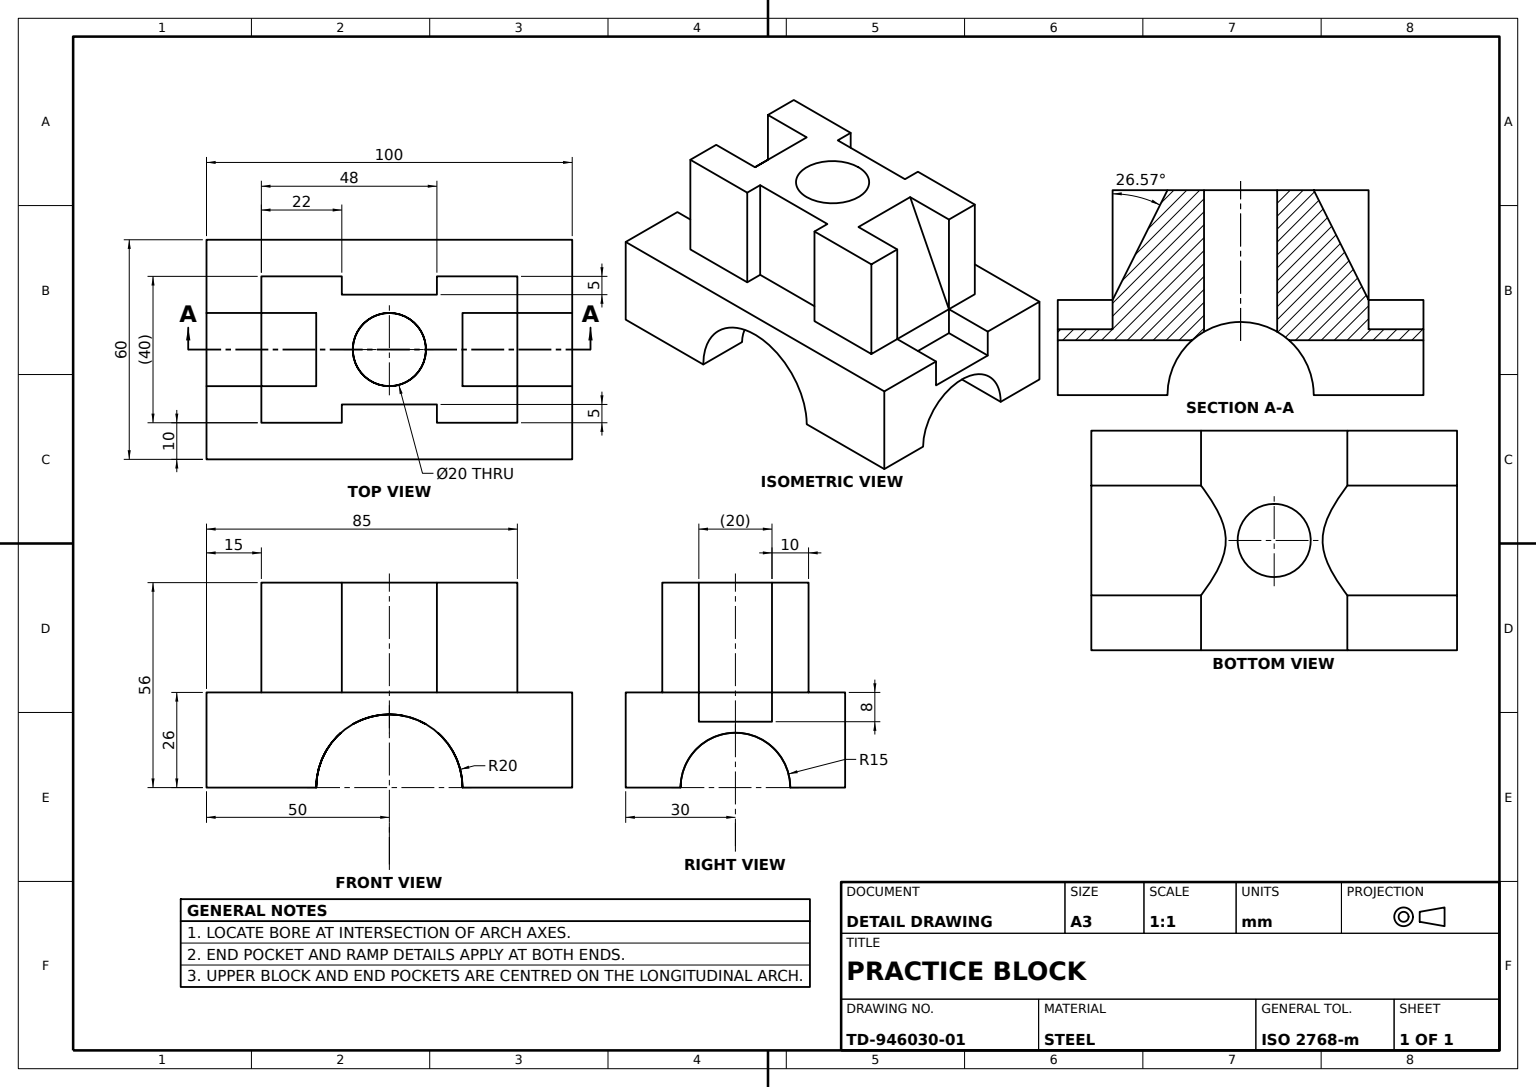
ISO-10303-21;
HEADER;
FILE_DESCRIPTION((''),'2;1');
FILE_NAME('','',(''),(''),'','','');
FILE_SCHEMA(('AUTOMOTIVE_DESIGN'));
ENDSEC;
DATA;
#1=APPLICATION_CONTEXT('');
#2=PRODUCT_CONTEXT('',#1,'mechanical');
#3=PRODUCT('','','',(#2));
#4=PRODUCT_DEFINITION_FORMATION('','',#3);
#5=PRODUCT_DEFINITION_CONTEXT('',#1,'design');
#6=PRODUCT_DEFINITION('','',#4,#5);
#7=PRODUCT_DEFINITION_SHAPE('','',#6);
#8=(LENGTH_UNIT()NAMED_UNIT(*)SI_UNIT(.MILLI.,.METRE.));
#9=(NAMED_UNIT(*)PLANE_ANGLE_UNIT()SI_UNIT($,.RADIAN.));
#10=(NAMED_UNIT(*)SI_UNIT($,.STERADIAN.)SOLID_ANGLE_UNIT());
#11=UNCERTAINTY_MEASURE_WITH_UNIT(LENGTH_MEASURE(1.E-05),#8,'distance_accuracy_value','');
#12=(GEOMETRIC_REPRESENTATION_CONTEXT(3)GLOBAL_UNCERTAINTY_ASSIGNED_CONTEXT((#11))GLOBAL_UNIT_ASSIGNED_CONTEXT((#8,#9,#10))REPRESENTATION_CONTEXT('',''));
#13=CARTESIAN_POINT('',(-20.,0.,15.));
#14=VERTEX_POINT('',#13);
#15=CARTESIAN_POINT('',(-20.,0.,30.));
#16=VERTEX_POINT('',#15);
#17=CARTESIAN_POINT('',(-20.,0.,91.));
#18=DIRECTION('',(0.,0.,1.));
#19=VECTOR('',#18,1000.);
#20=LINE('',#17,#19);
#21=EDGE_CURVE('',#14,#16,#20,.T.);
#22=ORIENTED_EDGE('',*,*,#21,.F.);
#23=CARTESIAN_POINT('',(-20.,0.,-15.));
#24=VERTEX_POINT('',#23);
#25=CARTESIAN_POINT('',(-20.,1.039988,-15.));
#26=CARTESIAN_POINT('',(-19.91945,2.055511,-14.89307));
#27=CARTESIAN_POINT('',(-19.68971,3.545099,-14.583876));
#28=CARTESIAN_POINT('',(-19.594347,4.038167,-14.455074));
#29=CARTESIAN_POINT('',(-19.370481,5.00297,-14.150132));
#30=CARTESIAN_POINT('',(-19.243229,5.47024,-13.975697));
#31=CARTESIAN_POINT('',(-18.961995,6.377158,-13.585856));
#32=CARTESIAN_POINT('',(-18.807998,6.816797,-13.37044));
#33=CARTESIAN_POINT('',(-18.476456,7.670078,-12.899895));
#34=CARTESIAN_POINT('',(-18.297983,8.085575,-12.64341));
#35=CARTESIAN_POINT('',(-17.739419,9.278133,-11.825632));
#36=CARTESIAN_POINT('',(-17.337061,10.001911,-11.218166));
#37=CARTESIAN_POINT('',(-16.711435,10.994586,-10.214717));
#38=CARTESIAN_POINT('',(-16.498395,11.31093,-9.863302));
#39=CARTESIAN_POINT('',(-16.073156,11.907469,-9.134223));
#40=CARTESIAN_POINT('',(-15.861739,12.18674,-8.758001));
#41=CARTESIAN_POINT('',(-15.238528,12.970461,-7.592364));
#42=CARTESIAN_POINT('',(-14.836864,13.421647,-6.766908));
#43=CARTESIAN_POINT('',(-14.29593,13.989091,-5.434909));
#44=CARTESIAN_POINT('',(-14.125386,14.160451,-4.972426));
#45=CARTESIAN_POINT('',(-13.822168,14.456576,-4.031229));
#46=CARTESIAN_POINT('',(-13.688686,14.582271,-3.550951));
#47=CARTESIAN_POINT('',(-13.467259,14.78701,-2.568307));
#48=CARTESIAN_POINT('',(-13.379218,14.866168,-2.065023));
#49=CARTESIAN_POINT('',(-13.259474,14.973069,-1.036579));
#50=CARTESIAN_POINT('',(-13.22921,14.9996,-0.523513));
#51=CARTESIAN_POINT('',(-13.228313,15.000391,0.500332));
#52=CARTESIAN_POINT('',(-13.257676,14.974649,1.011111));
#53=CARTESIAN_POINT('',(-13.374088,14.870772,2.030418));
#54=CARTESIAN_POINT('',(-13.461925,14.791862,2.540716));
#55=CARTESIAN_POINT('',(-13.682828,14.587763,3.528684));
#56=CARTESIAN_POINT('',(-13.816081,14.462383,4.010379));
#57=CARTESIAN_POINT('',(-14.118367,14.167438,4.952509));
#58=CARTESIAN_POINT('',(-14.288407,13.996778,5.415214));
#59=CARTESIAN_POINT('',(-14.829898,13.429354,6.752021));
#60=CARTESIAN_POINT('',(-15.232138,12.977984,7.579673));
#61=CARTESIAN_POINT('',(-15.856074,12.194115,8.747768));
#62=CARTESIAN_POINT('',(-16.067715,11.914813,9.124663));
#63=CARTESIAN_POINT('',(-16.493336,11.318308,9.854854));
#64=CARTESIAN_POINT('',(-16.706461,11.002121,10.206576));
#65=CARTESIAN_POINT('',(-17.331547,10.011365,11.209639));
#66=CARTESIAN_POINT('',(-17.73267,9.290466,11.815456));
#67=CARTESIAN_POINT('',(-18.288634,8.106539,12.629864));
#68=CARTESIAN_POINT('',(-18.466869,7.693327,12.886183));
#69=CARTESIAN_POINT('',(-18.801726,6.834298,13.361638));
#70=CARTESIAN_POINT('',(-18.956617,6.393125,13.578352));
#71=CARTESIAN_POINT('',(-19.238591,5.486526,13.969314));
#72=CARTESIAN_POINT('',(-19.365686,5.021105,14.143566));
#73=CARTESIAN_POINT('',(-19.588837,4.064329,14.447602));
#74=CARTESIAN_POINT('',(-19.685272,3.570495,14.57789));
#75=CARTESIAN_POINT('',(-19.91921,2.063634,14.892772));
#76=CARTESIAN_POINT('',(-20.,1.041225,15.));
#77=B_SPLINE_CURVE_WITH_KNOTS('',3,(#23,#25,#26,#27,#28,#29,#30,#31,#32,#33,#34,#35,#36,#37,#38,#39,#40,#41,#42,#43,#44,#45,#46,#47,#48,#49,#50,#51,#52,#53,#54,#55,#56,#57,#58,#59,#60,#61,#62,#63,#64,#65,#66,#67,#68,#69,#70,#71,#72,#73,#74,#75,#76,#13),.UNSPECIFIED.,.F.,.F.,(4,2,2,2,2,2,2,2,2,2,2,2,2,2,2,2,2,2,2,2,2,2,2,2,2,2,4),(0.,0.003069136,0.004603704,0.006138272,0.00767284,0.009207408,0.012276544,0.013811112,0.01534568,0.018414816,0.019949384,0.021483952,0.02301852,0.024553088,0.026087656,0.027622224,0.029156792,0.03069136,0.033760496,0.035295064,0.036829632,0.039898768,0.041433336,0.042967904,0.044502472,0.04603704,0.049106176),.UNSPECIFIED.);
#78=EDGE_CURVE('',#24,#14,#77,.T.);
#79=ORIENTED_EDGE('',*,*,#78,.F.);
#80=CARTESIAN_POINT('',(-20.,0.,-30.));
#81=VERTEX_POINT('',#80);
#82=EDGE_CURVE('',#81,#24,#20,.T.);
#83=ORIENTED_EDGE('',*,*,#82,.F.);
#84=CARTESIAN_POINT('',(20.,0.,-30.));
#85=VERTEX_POINT('',#84);
#86=CARTESIAN_POINT('',(0.,0.,-30.));
#87=DIRECTION('',(0.,0.,-1.));
#88=DIRECTION('',(-1.,0.,0.));
#89=AXIS2_PLACEMENT_3D('',#86,#87,#88);
#90=CIRCLE('',#89,20.);
#91=EDGE_CURVE('',#81,#85,#90,.T.);
#92=ORIENTED_EDGE('',*,*,#91,.T.);
#93=CARTESIAN_POINT('',(20.,0.,-15.));
#94=VERTEX_POINT('',#93);
#95=CARTESIAN_POINT('',(20.,0.,91.));
#96=VECTOR('',#87,1000.);
#97=LINE('',#95,#96);
#98=EDGE_CURVE('',#94,#85,#97,.T.);
#99=ORIENTED_EDGE('',*,*,#98,.F.);
#100=CARTESIAN_POINT('',(20.,0.,15.));
#101=VERTEX_POINT('',#100);
#102=CARTESIAN_POINT('',(20.,1.039988,15.));
#103=CARTESIAN_POINT('',(19.91945,2.055511,14.89307));
#104=CARTESIAN_POINT('',(19.68971,3.545099,14.583876));
#105=CARTESIAN_POINT('',(19.594347,4.038167,14.455074));
#106=CARTESIAN_POINT('',(19.370481,5.00297,14.150132));
#107=CARTESIAN_POINT('',(19.243229,5.47024,13.975697));
#108=CARTESIAN_POINT('',(18.961995,6.377158,13.585856));
#109=CARTESIAN_POINT('',(18.807998,6.816797,13.37044));
#110=CARTESIAN_POINT('',(18.476456,7.670078,12.899895));
#111=CARTESIAN_POINT('',(18.297983,8.085575,12.64341));
#112=CARTESIAN_POINT('',(17.739419,9.278133,11.825632));
#113=CARTESIAN_POINT('',(17.337061,10.001911,11.218166));
#114=CARTESIAN_POINT('',(16.711435,10.994586,10.214717));
#115=CARTESIAN_POINT('',(16.498395,11.31093,9.863302));
#116=CARTESIAN_POINT('',(16.073156,11.907469,9.134223));
#117=CARTESIAN_POINT('',(15.861739,12.18674,8.758001));
#118=CARTESIAN_POINT('',(15.238528,12.970461,7.592364));
#119=CARTESIAN_POINT('',(14.836864,13.421647,6.766908));
#120=CARTESIAN_POINT('',(14.29593,13.989091,5.434909));
#121=CARTESIAN_POINT('',(14.125386,14.160451,4.972426));
#122=CARTESIAN_POINT('',(13.822168,14.456576,4.031229));
#123=CARTESIAN_POINT('',(13.688686,14.582271,3.550951));
#124=CARTESIAN_POINT('',(13.467259,14.78701,2.568307));
#125=CARTESIAN_POINT('',(13.379218,14.866168,2.065023));
#126=CARTESIAN_POINT('',(13.259474,14.973069,1.036579));
#127=CARTESIAN_POINT('',(13.22921,14.9996,0.523513));
#128=CARTESIAN_POINT('',(13.228313,15.000391,-0.500332));
#129=CARTESIAN_POINT('',(13.257676,14.974649,-1.011111));
#130=CARTESIAN_POINT('',(13.374088,14.870772,-2.030418));
#131=CARTESIAN_POINT('',(13.461925,14.791862,-2.540716));
#132=CARTESIAN_POINT('',(13.682828,14.587763,-3.528684));
#133=CARTESIAN_POINT('',(13.816081,14.462383,-4.010379));
#134=CARTESIAN_POINT('',(14.118367,14.167438,-4.952509));
#135=CARTESIAN_POINT('',(14.288407,13.996778,-5.415214));
#136=CARTESIAN_POINT('',(14.829898,13.429354,-6.752021));
#137=CARTESIAN_POINT('',(15.232138,12.977984,-7.579673));
#138=CARTESIAN_POINT('',(15.856074,12.194115,-8.747768));
#139=CARTESIAN_POINT('',(16.067715,11.914813,-9.124663));
#140=CARTESIAN_POINT('',(16.493336,11.318308,-9.854854));
#141=CARTESIAN_POINT('',(16.706461,11.002121,-10.206576));
#142=CARTESIAN_POINT('',(17.331547,10.011365,-11.209639));
#143=CARTESIAN_POINT('',(17.73267,9.290466,-11.815456));
#144=CARTESIAN_POINT('',(18.288634,8.106539,-12.629864));
#145=CARTESIAN_POINT('',(18.466869,7.693327,-12.886183));
#146=CARTESIAN_POINT('',(18.801726,6.834298,-13.361638));
#147=CARTESIAN_POINT('',(18.956617,6.393125,-13.578352));
#148=CARTESIAN_POINT('',(19.238591,5.486526,-13.969314));
#149=CARTESIAN_POINT('',(19.365686,5.021105,-14.143566));
#150=CARTESIAN_POINT('',(19.588837,4.064329,-14.447602));
#151=CARTESIAN_POINT('',(19.685272,3.570495,-14.57789));
#152=CARTESIAN_POINT('',(19.91921,2.063634,-14.892772));
#153=CARTESIAN_POINT('',(20.,1.041225,-15.));
#154=B_SPLINE_CURVE_WITH_KNOTS('',3,(#100,#102,#103,#104,#105,#106,#107,#108,#109,#110,#111,#112,#113,#114,#115,#116,#117,#118,#119,#120,#121,#122,#123,#124,#125,#126,#127,#128,#129,#130,#131,#132,#133,#134,#135,#136,#137,#138,#139,#140,#141,#142,#143,#144,#145,#146,#147,#148,#149,#150,#151,#152,#153,#93),.UNSPECIFIED.,.F.,.F.,(4,2,2,2,2,2,2,2,2,2,2,2,2,2,2,2,2,2,2,2,2,2,2,2,2,2,4),(0.,0.003069136,0.004603704,0.006138272,0.00767284,0.009207408,0.012276544,0.013811112,0.01534568,0.018414816,0.019949384,0.021483952,0.02301852,0.024553088,0.026087656,0.027622224,0.029156792,0.03069136,0.033760496,0.035295064,0.036829632,0.039898768,0.041433336,0.042967904,0.044502472,0.04603704,0.049106176),.UNSPECIFIED.);
#155=EDGE_CURVE('',#101,#94,#154,.T.);
#156=ORIENTED_EDGE('',*,*,#155,.F.);
#157=CARTESIAN_POINT('',(20.,0.,30.));
#158=VERTEX_POINT('',#157);
#159=EDGE_CURVE('',#158,#101,#97,.T.);
#160=ORIENTED_EDGE('',*,*,#159,.F.);
#161=CARTESIAN_POINT('',(0.,0.,30.));
#162=AXIS2_PLACEMENT_3D('',#161,#87,#88);
#163=CIRCLE('',#162,20.);
#164=EDGE_CURVE('',#16,#158,#163,.T.);
#165=ORIENTED_EDGE('',*,*,#164,.F.);
#166=EDGE_LOOP('',(#22,#79,#83,#92,#99,#156,#160,#165));
#167=FACE_OUTER_BOUND('',#166,.T.);
#168=CARTESIAN_POINT('',(0.,20.,-10.));
#169=VERTEX_POINT('',#168);
#170=CARTESIAN_POINT('',(0.,20.,10.));
#171=VERTEX_POINT('',#170);
#172=CARTESIAN_POINT('',(0.662824,20.,-10.));
#173=CARTESIAN_POINT('',(1.337358,19.96586,-9.932201));
#174=CARTESIAN_POINT('',(2.633374,19.836568,-9.669668));
#175=CARTESIAN_POINT('',(3.261651,19.742012,-9.476181));
#176=CARTESIAN_POINT('',(4.479828,19.501707,-8.964793));
#177=CARTESIAN_POINT('',(5.051691,19.359535,-8.654336));
#178=CARTESIAN_POINT('',(5.85513,19.125774,-8.113059));
#179=CARTESIAN_POINT('',(6.114055,19.044367,-7.919815));
#180=CARTESIAN_POINT('',(6.614275,18.876466,-7.507097));
#181=CARTESIAN_POINT('',(6.854053,18.790445,-7.288703));
#182=CARTESIAN_POINT('',(7.5347,18.532774,-6.606153));
#183=CARTESIAN_POINT('',(7.941207,18.360117,-6.111817));
#184=CARTESIAN_POINT('',(8.481335,18.1137,-5.307657));
#185=CARTESIAN_POINT('',(8.650477,18.033267,-5.027419));
#186=CARTESIAN_POINT('',(8.958743,17.882125,-4.454953));
#187=CARTESIAN_POINT('',(9.09831,17.811251,-4.162427));
#188=CARTESIAN_POINT('',(9.473971,17.616002,-3.265589));
#189=CARTESIAN_POINT('',(9.667555,17.508897,-2.642228));
#190=CARTESIAN_POINT('',(9.866225,17.397223,-1.663837));
#191=CARTESIAN_POINT('',(9.916444,17.368524,-1.331983));
#192=CARTESIAN_POINT('',(9.982916,17.330403,-0.671885));
#193=CARTESIAN_POINT('',(10.016356,17.311033,-0.011145));
#194=CARTESIAN_POINT('',(9.984348,17.329576,0.650875));
#195=CARTESIAN_POINT('',(9.918944,17.367094,1.313545));
#196=CARTESIAN_POINT('',(9.869061,17.395611,1.646751));
#197=CARTESIAN_POINT('',(9.672697,17.506042,2.622893));
#198=CARTESIAN_POINT('',(9.479948,17.612826,3.249621));
#199=CARTESIAN_POINT('',(9.101073,17.80985,4.156662));
#200=CARTESIAN_POINT('',(8.959157,17.881917,4.454122));
#201=CARTESIAN_POINT('',(8.650923,18.033053,5.026653));
#202=CARTESIAN_POINT('',(8.484067,18.112413,5.303235));
#203=CARTESIAN_POINT('',(8.1253,18.27617,5.838081));
#204=CARTESIAN_POINT('',(7.933387,18.360572,6.096344));
#205=CARTESIAN_POINT('',(7.524023,18.532089,6.594931));
#206=CARTESIAN_POINT('',(7.305468,18.619601,6.836244));
#207=CARTESIAN_POINT('',(6.621674,18.878321,7.521291));
#208=CARTESIAN_POINT('',(6.127019,19.046527,7.929448));
#209=CARTESIAN_POINT('',(5.324467,19.280241,8.470784));
#210=CARTESIAN_POINT('',(5.046779,19.355059,8.63931));
#211=CARTESIAN_POINT('',(4.469638,19.496425,8.951535));
#212=CARTESIAN_POINT('',(4.173386,19.562132,9.093376));
#213=CARTESIAN_POINT('',(3.270148,19.740386,9.472734));
#214=CARTESIAN_POINT('',(2.645303,19.835018,9.666499));
#215=CARTESIAN_POINT('',(1.671635,19.932688,9.864854));
#216=CARTESIAN_POINT('',(1.33927,19.957906,9.915588));
#217=CARTESIAN_POINT('',(0.67177,19.991508,9.983048));
#218=CARTESIAN_POINT('',(0.335902,20.,10.));
#219=B_SPLINE_CURVE_WITH_KNOTS('',3,(#168,#172,#173,#174,#175,#176,#177,#178,#179,#180,#181,#182,#183,#184,#185,#186,#187,#188,#189,#190,#191,#192,#193,#194,#195,#196,#197,#198,#199,#200,#201,#202,#203,#204,#205,#206,#207,#208,#209,#210,#211,#212,#213,#214,#215,#216,#217,#218,#170),.UNSPECIFIED.,.F.,.F.,(4,2,2,2,2,2,2,2,2,2,2,1,2,2,2,2,2,2,2,2,2,2,2,2,4),(0.031809829,0.033794481,0.035779133,0.037763785,0.038756111,0.039748437,0.041733089,0.042725415,0.043717741,0.045702393,0.046694719,0.047687045,0.048679371,0.049671697,0.051656349,0.052648675,0.053641001,0.054633327,0.055625653,0.057610305,0.058602631,0.059594957,0.061579609,0.062571935,0.063564261),.UNSPECIFIED.);
#220=EDGE_CURVE('',#169,#171,#219,.T.);
#221=ORIENTED_EDGE('',*,*,#220,.F.);
#222=CARTESIAN_POINT('',(-0.672977,20.,10.));
#223=CARTESIAN_POINT('',(-1.332651,19.966148,9.932775));
#224=CARTESIAN_POINT('',(-2.303481,19.869568,9.736682));
#225=CARTESIAN_POINT('',(-2.623955,19.82972,9.655314));
#226=CARTESIAN_POINT('',(-3.258595,19.735361,9.46001));
#227=CARTESIAN_POINT('',(-3.570245,19.68116,9.346688));
#228=CARTESIAN_POINT('',(-4.47599,19.502418,8.966294));
#229=CARTESIAN_POINT('',(-5.046758,19.360939,8.657561));
#230=CARTESIAN_POINT('',(-5.856049,19.125523,8.112488));
#231=CARTESIAN_POINT('',(-6.117628,19.043201,7.916989));
#232=CARTESIAN_POINT('',(-6.615216,18.876117,7.506198));
#233=CARTESIAN_POINT('',(-6.85263,18.790958,7.290011));
#234=CARTESIAN_POINT('',(-7.305528,18.619556,6.836084));
#235=CARTESIAN_POINT('',(-7.521012,18.533309,6.598346));
#236=CARTESIAN_POINT('',(-7.930131,18.361977,6.100559));
#237=CARTESIAN_POINT('',(-8.124688,18.276454,5.839036));
#238=CARTESIAN_POINT('',(-8.665899,18.029407,5.032076));
#239=CARTESIAN_POINT('',(-8.971565,17.87711,4.464615));
#240=CARTESIAN_POINT('',(-9.348137,17.681412,3.566198));
#241=CARTESIAN_POINT('',(-9.459893,17.621654,3.258795));
#242=CARTESIAN_POINT('',(-9.654487,17.515797,2.626821));
#243=CARTESIAN_POINT('',(-9.736776,17.469998,2.303114));
#244=CARTESIAN_POINT('',(-9.932947,17.359697,1.331598));
#245=CARTESIAN_POINT('',(-9.999352,17.320882,0.67518));
#246=CARTESIAN_POINT('',(-10.000317,17.320325,-0.323101));
#247=CARTESIAN_POINT('',(-9.983759,17.329917,-0.660503));
#248=CARTESIAN_POINT('',(-9.917374,17.367992,-1.32567));
#249=CARTESIAN_POINT('',(-9.867851,17.396296,-1.653624));
#250=CARTESIAN_POINT('',(-9.737328,17.469689,-2.300737));
#251=CARTESIAN_POINT('',(-9.656326,17.514779,-2.619897));
#252=CARTESIAN_POINT('',(-9.462991,17.619986,-3.249662));
#253=CARTESIAN_POINT('',(-9.349903,17.68049,-3.561881));
#254=CARTESIAN_POINT('',(-8.969437,17.878225,-4.469897));
#255=CARTESIAN_POINT('',(-8.661621,18.031458,-5.039316));
#256=CARTESIAN_POINT('',(-8.120596,18.278272,-5.8447));
#257=CARTESIAN_POINT('',(-7.925877,18.363827,-6.106151));
#258=CARTESIAN_POINT('',(-7.514756,18.53586,-6.605531));
#259=CARTESIAN_POINT('',(-7.298535,18.622304,-6.843559));
#260=CARTESIAN_POINT('',(-6.618065,18.879524,-7.524153));
#261=CARTESIAN_POINT('',(-6.122388,19.048215,-7.933625));
#262=CARTESIAN_POINT('',(-5.039143,19.362984,-8.662164));
#263=CARTESIAN_POINT('',(-4.465604,19.504685,-8.97118));
#264=CARTESIAN_POINT('',(-3.565122,19.68206,-9.348574));
#265=CARTESIAN_POINT('',(-3.257761,19.73546,-9.460211));
#266=CARTESIAN_POINT('',(-2.627882,19.829161,-9.654161));
#267=CARTESIAN_POINT('',(-2.30313,19.869661,-9.736875));
#268=CARTESIAN_POINT('',(-1.322767,19.967014,-9.934526));
#269=CARTESIAN_POINT('',(-0.66398,20.,-10.));
#270=B_SPLINE_CURVE_WITH_KNOTS('',3,(#170,#222,#223,#224,#225,#226,#227,#228,#229,#230,#231,#232,#233,#234,#235,#236,#237,#238,#239,#240,#241,#242,#243,#244,#245,#246,#247,#248,#249,#250,#251,#252,#253,#254,#255,#256,#257,#258,#259,#260,#261,#262,#263,#264,#265,#266,#267,#268,#269,#168),.UNSPECIFIED.,.F.,.F.,(4,2,2,2,2,2,2,2,2,2,2,2,2,2,2,2,2,2,2,2,2,2,2,2,4),(0.,0.001988114,0.002982171,0.003976229,0.005964343,0.0069584,0.007952457,0.008946514,0.009940571,0.011928686,0.012922743,0.0139168,0.015904914,0.016898971,0.017893029,0.018887086,0.019881143,0.021869257,0.022863314,0.023857371,0.025845486,0.0278336,0.028827657,0.029821714,0.031809829),.UNSPECIFIED.);
#271=EDGE_CURVE('',#171,#169,#270,.T.);
#272=ORIENTED_EDGE('',*,*,#271,.F.);
#273=EDGE_LOOP('',(#221,#272));
#274=FACE_BOUND('',#273,.T.);
#275=CARTESIAN_POINT('',(0.,0.,91.));
#276=AXIS2_PLACEMENT_3D('',#275,#87,#88);
#277=CYLINDRICAL_SURFACE('',#276,20.);
#278=ADVANCED_FACE('',(#167,#274),#277,.F.);
#279=CARTESIAN_POINT('',(20.,56.,-10.));
#280=VERTEX_POINT('',#279);
#281=CARTESIAN_POINT('',(20.,56.,10.));
#282=VERTEX_POINT('',#281);
#283=LINE('',#279,#19);
#284=EDGE_CURVE('',#280,#282,#283,.T.);
#285=ORIENTED_EDGE('',*,*,#284,.T.);
#286=CARTESIAN_POINT('',(35.,26.,10.));
#287=VERTEX_POINT('',#286);
#288=DIRECTION('',(-0.447213595,0.894427191,0.));
#289=VECTOR('',#288,1000.);
#290=LINE('',#281,#289);
#291=EDGE_CURVE('',#287,#282,#290,.T.);
#292=ORIENTED_EDGE('',*,*,#291,.F.);
#293=CARTESIAN_POINT('',(35.,26.,-10.));
#294=VERTEX_POINT('',#293);
#295=LINE('',#293,#19);
#296=EDGE_CURVE('',#294,#287,#295,.T.);
#297=ORIENTED_EDGE('',*,*,#296,.F.);
#298=LINE('',#279,#289);
#299=EDGE_CURVE('',#294,#280,#298,.T.);
#300=ORIENTED_EDGE('',*,*,#299,.T.);
#301=EDGE_LOOP('',(#285,#292,#297,#300));
#302=FACE_OUTER_BOUND('',#301,.T.);
#303=DIRECTION('',(0.894427191,0.447213595,0.));
#304=AXIS2_PLACEMENT_3D('',#279,#303,#288);
#305=PLANE('',#304);
#306=ADVANCED_FACE('',(#302),#305,.T.);
#307=CARTESIAN_POINT('',(35.,56.,-20.));
#308=VERTEX_POINT('',#307);
#309=CARTESIAN_POINT('',(35.,26.,-20.));
#310=VERTEX_POINT('',#309);
#311=DIRECTION('',(0.,-1.,0.));
#312=VECTOR('',#311,1000.);
#313=LINE('',#307,#312);
#314=EDGE_CURVE('',#308,#310,#313,.T.);
#315=ORIENTED_EDGE('',*,*,#314,.T.);
#316=CARTESIAN_POINT('',(13.,26.,-20.));
#317=VERTEX_POINT('',#316);
#318=VECTOR('',#88,1000.);
#319=LINE('',#309,#318);
#320=EDGE_CURVE('',#310,#317,#319,.T.);
#321=ORIENTED_EDGE('',*,*,#320,.T.);
#322=CARTESIAN_POINT('',(13.,56.,-20.));
#323=VERTEX_POINT('',#322);
#324=DIRECTION('',(0.,1.,0.));
#325=VECTOR('',#324,1000.);
#326=LINE('',#316,#325);
#327=EDGE_CURVE('',#317,#323,#326,.T.);
#328=ORIENTED_EDGE('',*,*,#327,.T.);
#329=LINE('',#307,#318);
#330=EDGE_CURVE('',#308,#323,#329,.T.);
#331=ORIENTED_EDGE('',*,*,#330,.F.);
#332=EDGE_LOOP('',(#315,#321,#328,#331));
#333=FACE_OUTER_BOUND('',#332,.T.);
#334=DIRECTION('',(1.,0.,0.));
#335=AXIS2_PLACEMENT_3D('',#307,#18,#334);
#336=PLANE('',#335);
#337=ADVANCED_FACE('',(#333),#336,.F.);
#338=CARTESIAN_POINT('',(-20.,56.,10.));
#339=VERTEX_POINT('',#338);
#340=CARTESIAN_POINT('',(-35.,26.,10.));
#341=VERTEX_POINT('',#340);
#342=DIRECTION('',(-0.447213595,-0.894427191,0.));
#343=VECTOR('',#342,1000.);
#344=LINE('',#338,#343);
#345=EDGE_CURVE('',#339,#341,#344,.T.);
#346=ORIENTED_EDGE('',*,*,#345,.F.);
#347=CARTESIAN_POINT('',(-20.,56.,-10.));
#348=VERTEX_POINT('',#347);
#349=LINE('',#338,#96);
#350=EDGE_CURVE('',#339,#348,#349,.T.);
#351=ORIENTED_EDGE('',*,*,#350,.T.);
#352=CARTESIAN_POINT('',(-35.,26.,-10.));
#353=VERTEX_POINT('',#352);
#354=LINE('',#347,#343);
#355=EDGE_CURVE('',#348,#353,#354,.T.);
#356=ORIENTED_EDGE('',*,*,#355,.T.);
#357=LINE('',#352,#19);
#358=EDGE_CURVE('',#353,#341,#357,.T.);
#359=ORIENTED_EDGE('',*,*,#358,.T.);
#360=EDGE_LOOP('',(#346,#351,#356,#359));
#361=FACE_OUTER_BOUND('',#360,.T.);
#362=DIRECTION('',(-0.894427191,0.447213595,0.));
#363=AXIS2_PLACEMENT_3D('',#347,#362,#342);
#364=PLANE('',#363);
#365=ADVANCED_FACE('',(#361),#364,.T.);
#366=CARTESIAN_POINT('',(35.,56.,-10.));
#367=VERTEX_POINT('',#366);
#368=LINE('',#366,#318);
#369=EDGE_CURVE('',#367,#280,#368,.T.);
#370=ORIENTED_EDGE('',*,*,#369,.T.);
#371=ORIENTED_EDGE('',*,*,#299,.F.);
#372=LINE('',#293,#325);
#373=EDGE_CURVE('',#294,#367,#372,.T.);
#374=ORIENTED_EDGE('',*,*,#373,.T.);
#375=EDGE_LOOP('',(#370,#371,#374));
#376=FACE_OUTER_BOUND('',#375,.T.);
#377=AXIS2_PLACEMENT_3D('',#293,#87,#88);
#378=PLANE('',#377);
#379=ADVANCED_FACE('',(#376),#378,.F.);
#380=CARTESIAN_POINT('',(35.,18.,10.));
#381=VERTEX_POINT('',#380);
#382=LINE('',#380,#325);
#383=EDGE_CURVE('',#381,#287,#382,.T.);
#384=ORIENTED_EDGE('',*,*,#383,.F.);
#385=CARTESIAN_POINT('',(35.,18.,-10.));
#386=VERTEX_POINT('',#385);
#387=LINE('',#380,#19);
#388=EDGE_CURVE('',#386,#381,#387,.T.);
#389=ORIENTED_EDGE('',*,*,#388,.F.);
#390=LINE('',#385,#325);
#391=EDGE_CURVE('',#386,#294,#390,.T.);
#392=ORIENTED_EDGE('',*,*,#391,.T.);
#393=ORIENTED_EDGE('',*,*,#296,.T.);
#394=EDGE_LOOP('',(#384,#389,#392,#393));
#395=FACE_OUTER_BOUND('',#394,.T.);
#396=AXIS2_PLACEMENT_3D('',#380,#88,#18);
#397=PLANE('',#396);
#398=ADVANCED_FACE('',(#395),#397,.F.);
#399=CARTESIAN_POINT('',(-35.,18.,10.));
#400=VERTEX_POINT('',#399);
#401=CARTESIAN_POINT('',(-35.,18.,-10.));
#402=VERTEX_POINT('',#401);
#403=LINE('',#399,#96);
#404=EDGE_CURVE('',#400,#402,#403,.T.);
#405=ORIENTED_EDGE('',*,*,#404,.F.);
#406=LINE('',#399,#325);
#407=EDGE_CURVE('',#400,#341,#406,.T.);
#408=ORIENTED_EDGE('',*,*,#407,.T.);
#409=ORIENTED_EDGE('',*,*,#358,.F.);
#410=LINE('',#401,#325);
#411=EDGE_CURVE('',#402,#353,#410,.T.);
#412=ORIENTED_EDGE('',*,*,#411,.F.);
#413=EDGE_LOOP('',(#405,#408,#409,#412));
#414=FACE_OUTER_BOUND('',#413,.T.);
#415=AXIS2_PLACEMENT_3D('',#399,#334,#87);
#416=PLANE('',#415);
#417=ADVANCED_FACE('',(#414),#416,.F.);
#418=CARTESIAN_POINT('',(50.,26.,-30.));
#419=VERTEX_POINT('',#418);
#420=CARTESIAN_POINT('',(-50.,26.,-30.));
#421=VERTEX_POINT('',#420);
#422=LINE('',#418,#318);
#423=EDGE_CURVE('',#419,#421,#422,.T.);
#424=ORIENTED_EDGE('',*,*,#423,.F.);
#425=CARTESIAN_POINT('',(50.,0.,-30.));
#426=VERTEX_POINT('',#425);
#427=LINE('',#418,#312);
#428=EDGE_CURVE('',#419,#426,#427,.T.);
#429=ORIENTED_EDGE('',*,*,#428,.T.);
#430=LINE('',#425,#318);
#431=EDGE_CURVE('',#426,#85,#430,.T.);
#432=ORIENTED_EDGE('',*,*,#431,.T.);
#433=ORIENTED_EDGE('',*,*,#91,.F.);
#434=CARTESIAN_POINT('',(-50.,0.,-30.));
#435=VERTEX_POINT('',#434);
#436=EDGE_CURVE('',#81,#435,#430,.T.);
#437=ORIENTED_EDGE('',*,*,#436,.T.);
#438=LINE('',#420,#312);
#439=EDGE_CURVE('',#421,#435,#438,.T.);
#440=ORIENTED_EDGE('',*,*,#439,.F.);
#441=EDGE_LOOP('',(#424,#429,#432,#433,#437,#440));
#442=FACE_OUTER_BOUND('',#441,.T.);
#443=AXIS2_PLACEMENT_3D('',#418,#18,#334);
#444=PLANE('',#443);
#445=ADVANCED_FACE('',(#442),#444,.F.);
#446=CARTESIAN_POINT('',(0.,56.,10.));
#447=VERTEX_POINT('',#446);
#448=CARTESIAN_POINT('',(0.,56.,-10.));
#449=VERTEX_POINT('',#448);
#450=CARTESIAN_POINT('',(0.,56.,0.));
#451=AXIS2_PLACEMENT_3D('',#450,#324,#18);
#452=CIRCLE('',#451,10.);
#453=EDGE_CURVE('',#447,#449,#452,.T.);
#454=ORIENTED_EDGE('',*,*,#453,.T.);
#455=CARTESIAN_POINT('',(0.,-27.,-10.));
#456=LINE('',#455,#325);
#457=EDGE_CURVE('',#169,#449,#456,.T.);
#458=ORIENTED_EDGE('',*,*,#457,.F.);
#459=ORIENTED_EDGE('',*,*,#220,.T.);
#460=CARTESIAN_POINT('',(0.,-27.,10.));
#461=LINE('',#460,#325);
#462=EDGE_CURVE('',#171,#447,#461,.T.);
#463=ORIENTED_EDGE('',*,*,#462,.T.);
#464=EDGE_LOOP('',(#454,#458,#459,#463));
#465=FACE_OUTER_BOUND('',#464,.T.);
#466=CARTESIAN_POINT('',(0.,-27.,0.));
#467=AXIS2_PLACEMENT_3D('',#466,#324,#18);
#468=CYLINDRICAL_SURFACE('',#467,10.);
#469=ADVANCED_FACE('',(#465),#468,.F.);
#470=CARTESIAN_POINT('',(50.,18.,-10.));
#471=VERTEX_POINT('',#470);
#472=LINE('',#385,#318);
#473=EDGE_CURVE('',#471,#386,#472,.T.);
#474=ORIENTED_EDGE('',*,*,#473,.F.);
#475=CARTESIAN_POINT('',(50.,26.,-10.));
#476=VERTEX_POINT('',#475);
#477=LINE('',#470,#325);
#478=EDGE_CURVE('',#471,#476,#477,.T.);
#479=ORIENTED_EDGE('',*,*,#478,.T.);
#480=LINE('',#293,#318);
#481=EDGE_CURVE('',#476,#294,#480,.T.);
#482=ORIENTED_EDGE('',*,*,#481,.T.);
#483=ORIENTED_EDGE('',*,*,#391,.F.);
#484=EDGE_LOOP('',(#474,#479,#482,#483));
#485=FACE_OUTER_BOUND('',#484,.T.);
#486=AXIS2_PLACEMENT_3D('',#385,#87,#88);
#487=PLANE('',#486);
#488=ADVANCED_FACE('',(#485),#487,.F.);
#489=CARTESIAN_POINT('',(-50.,18.,-10.));
#490=VERTEX_POINT('',#489);
#491=CARTESIAN_POINT('',(-50.,26.,-10.));
#492=VERTEX_POINT('',#491);
#493=LINE('',#489,#325);
#494=EDGE_CURVE('',#490,#492,#493,.T.);
#495=ORIENTED_EDGE('',*,*,#494,.F.);
#496=LINE('',#401,#318);
#497=EDGE_CURVE('',#402,#490,#496,.T.);
#498=ORIENTED_EDGE('',*,*,#497,.F.);
#499=ORIENTED_EDGE('',*,*,#411,.T.);
#500=LINE('',#352,#318);
#501=EDGE_CURVE('',#353,#492,#500,.T.);
#502=ORIENTED_EDGE('',*,*,#501,.T.);
#503=EDGE_LOOP('',(#495,#498,#499,#502));
#504=FACE_OUTER_BOUND('',#503,.T.);
#505=AXIS2_PLACEMENT_3D('',#401,#87,#88);
#506=PLANE('',#505);
#507=ADVANCED_FACE('',(#504),#506,.F.);
#508=CARTESIAN_POINT('',(-13.,26.,-15.));
#509=VERTEX_POINT('',#508);
#510=CARTESIAN_POINT('',(13.,26.,-15.));
#511=VERTEX_POINT('',#510);
#512=VECTOR('',#334,1000.);
#513=LINE('',#508,#512);
#514=EDGE_CURVE('',#509,#511,#513,.T.);
#515=ORIENTED_EDGE('',*,*,#514,.F.);
#516=CARTESIAN_POINT('',(-13.,56.,-15.));
#517=VERTEX_POINT('',#516);
#518=LINE('',#508,#325);
#519=EDGE_CURVE('',#509,#517,#518,.T.);
#520=ORIENTED_EDGE('',*,*,#519,.T.);
#521=CARTESIAN_POINT('',(13.,56.,-15.));
#522=VERTEX_POINT('',#521);
#523=LINE('',#516,#512);
#524=EDGE_CURVE('',#517,#522,#523,.T.);
#525=ORIENTED_EDGE('',*,*,#524,.T.);
#526=LINE('',#510,#325);
#527=EDGE_CURVE('',#511,#522,#526,.T.);
#528=ORIENTED_EDGE('',*,*,#527,.F.);
#529=EDGE_LOOP('',(#515,#520,#525,#528));
#530=FACE_OUTER_BOUND('',#529,.T.);
#531=AXIS2_PLACEMENT_3D('',#508,#18,#334);
#532=PLANE('',#531);
#533=ADVANCED_FACE('',(#530),#532,.F.);
#534=CARTESIAN_POINT('',(-13.,26.,20.));
#535=VERTEX_POINT('',#534);
#536=CARTESIAN_POINT('',(-13.,56.,20.));
#537=VERTEX_POINT('',#536);
#538=LINE('',#534,#325);
#539=EDGE_CURVE('',#535,#537,#538,.T.);
#540=ORIENTED_EDGE('',*,*,#539,.F.);
#541=CARTESIAN_POINT('',(-13.,26.,15.));
#542=VERTEX_POINT('',#541);
#543=LINE('',#541,#19);
#544=EDGE_CURVE('',#542,#535,#543,.T.);
#545=ORIENTED_EDGE('',*,*,#544,.F.);
#546=CARTESIAN_POINT('',(-13.,56.,15.));
#547=VERTEX_POINT('',#546);
#548=LINE('',#541,#325);
#549=EDGE_CURVE('',#542,#547,#548,.T.);
#550=ORIENTED_EDGE('',*,*,#549,.T.);
#551=LINE('',#546,#19);
#552=EDGE_CURVE('',#547,#537,#551,.T.);
#553=ORIENTED_EDGE('',*,*,#552,.T.);
#554=EDGE_LOOP('',(#540,#545,#550,#553));
#555=FACE_OUTER_BOUND('',#554,.T.);
#556=AXIS2_PLACEMENT_3D('',#541,#88,#18);
#557=PLANE('',#556);
#558=ADVANCED_FACE('',(#555),#557,.F.);
#559=ORIENTED_EDGE('',*,*,#164,.T.);
#560=CARTESIAN_POINT('',(50.,0.,30.));
#561=VERTEX_POINT('',#560);
#562=CARTESIAN_POINT('',(-50.,0.,30.));
#563=LINE('',#562,#512);
#564=EDGE_CURVE('',#158,#561,#563,.T.);
#565=ORIENTED_EDGE('',*,*,#564,.T.);
#566=CARTESIAN_POINT('',(50.,26.,30.));
#567=VERTEX_POINT('',#566);
#568=LINE('',#566,#312);
#569=EDGE_CURVE('',#567,#561,#568,.T.);
#570=ORIENTED_EDGE('',*,*,#569,.F.);
#571=CARTESIAN_POINT('',(-50.,26.,30.));
#572=VERTEX_POINT('',#571);
#573=LINE('',#571,#512);
#574=EDGE_CURVE('',#572,#567,#573,.T.);
#575=ORIENTED_EDGE('',*,*,#574,.F.);
#576=VERTEX_POINT('',#562);
#577=LINE('',#571,#312);
#578=EDGE_CURVE('',#572,#576,#577,.T.);
#579=ORIENTED_EDGE('',*,*,#578,.T.);
#580=EDGE_CURVE('',#576,#16,#563,.T.);
#581=ORIENTED_EDGE('',*,*,#580,.T.);
#582=EDGE_LOOP('',(#559,#565,#570,#575,#579,#581));
#583=FACE_OUTER_BOUND('',#582,.T.);
#584=AXIS2_PLACEMENT_3D('',#571,#87,#88);
#585=PLANE('',#584);
#586=ADVANCED_FACE('',(#583),#585,.F.);
#587=LINE('',#510,#96);
#588=EDGE_CURVE('',#511,#317,#587,.T.);
#589=ORIENTED_EDGE('',*,*,#588,.F.);
#590=ORIENTED_EDGE('',*,*,#527,.T.);
#591=LINE('',#521,#96);
#592=EDGE_CURVE('',#522,#323,#591,.T.);
#593=ORIENTED_EDGE('',*,*,#592,.T.);
#594=ORIENTED_EDGE('',*,*,#327,.F.);
#595=EDGE_LOOP('',(#589,#590,#593,#594));
#596=FACE_OUTER_BOUND('',#595,.T.);
#597=AXIS2_PLACEMENT_3D('',#510,#334,#87);
#598=PLANE('',#597);
#599=ADVANCED_FACE('',(#596),#598,.F.);
#600=CARTESIAN_POINT('',(50.,0.,15.));
#601=VERTEX_POINT('',#600);
#602=CARTESIAN_POINT('',(71.,0.,15.));
#603=LINE('',#602,#318);
#604=EDGE_CURVE('',#601,#101,#603,.T.);
#605=ORIENTED_EDGE('',*,*,#604,.F.);
#606=CARTESIAN_POINT('',(50.,0.,0.));
#607=LINE('',#606,#96);
#608=EDGE_CURVE('',#561,#601,#607,.T.);
#609=ORIENTED_EDGE('',*,*,#608,.F.);
#610=ORIENTED_EDGE('',*,*,#564,.F.);
#611=ORIENTED_EDGE('',*,*,#159,.T.);
#612=EDGE_LOOP('',(#605,#609,#610,#611));
#613=FACE_OUTER_BOUND('',#612,.T.);
#614=CARTESIAN_POINT('',(0.,0.,0.));
#615=AXIS2_PLACEMENT_3D('',#614,#324,#18);
#616=PLANE('',#615);
#617=ADVANCED_FACE('',(#613),#616,.F.);
#618=ORIENTED_EDGE('',*,*,#82,.T.);
#619=CARTESIAN_POINT('',(-50.,0.,-15.));
#620=VERTEX_POINT('',#619);
#621=CARTESIAN_POINT('',(71.,0.,-15.));
#622=LINE('',#621,#318);
#623=EDGE_CURVE('',#24,#620,#622,.T.);
#624=ORIENTED_EDGE('',*,*,#623,.T.);
#625=LINE('',#434,#19);
#626=EDGE_CURVE('',#435,#620,#625,.T.);
#627=ORIENTED_EDGE('',*,*,#626,.F.);
#628=ORIENTED_EDGE('',*,*,#436,.F.);
#629=EDGE_LOOP('',(#618,#624,#627,#628));
#630=FACE_OUTER_BOUND('',#629,.T.);
#631=ADVANCED_FACE('',(#630),#616,.F.);
#632=ORIENTED_EDGE('',*,*,#388,.T.);
#633=CARTESIAN_POINT('',(50.,18.,10.));
#634=VERTEX_POINT('',#633);
#635=LINE('',#633,#512);
#636=EDGE_CURVE('',#381,#634,#635,.T.);
#637=ORIENTED_EDGE('',*,*,#636,.T.);
#638=LINE('',#470,#96);
#639=EDGE_CURVE('',#634,#471,#638,.T.);
#640=ORIENTED_EDGE('',*,*,#639,.T.);
#641=ORIENTED_EDGE('',*,*,#473,.T.);
#642=EDGE_LOOP('',(#632,#637,#640,#641));
#643=FACE_OUTER_BOUND('',#642,.T.);
#644=CARTESIAN_POINT('',(0.,18.,0.));
#645=AXIS2_PLACEMENT_3D('',#644,#311,#87);
#646=PLANE('',#645);
#647=ADVANCED_FACE('',(#643),#646,.F.);
#648=ORIENTED_EDGE('',*,*,#623,.F.);
#649=ORIENTED_EDGE('',*,*,#78,.T.);
#650=CARTESIAN_POINT('',(-50.,0.,15.));
#651=VERTEX_POINT('',#650);
#652=EDGE_CURVE('',#14,#651,#603,.T.);
#653=ORIENTED_EDGE('',*,*,#652,.T.);
#654=CARTESIAN_POINT('',(-50.,0.,0.));
#655=AXIS2_PLACEMENT_3D('',#654,#88,#18);
#656=CIRCLE('',#655,15.);
#657=EDGE_CURVE('',#651,#620,#656,.T.);
#658=ORIENTED_EDGE('',*,*,#657,.T.);
#659=EDGE_LOOP('',(#648,#649,#653,#658));
#660=FACE_OUTER_BOUND('',#659,.T.);
#661=CARTESIAN_POINT('',(71.,0.,0.));
#662=AXIS2_PLACEMENT_3D('',#661,#88,#18);
#663=CYLINDRICAL_SURFACE('',#662,15.);
#664=ADVANCED_FACE('',(#660),#663,.F.);
#665=CARTESIAN_POINT('',(-50.,18.,10.));
#666=VERTEX_POINT('',#665);
#667=LINE('',#665,#512);
#668=EDGE_CURVE('',#666,#400,#667,.T.);
#669=ORIENTED_EDGE('',*,*,#668,.T.);
#670=ORIENTED_EDGE('',*,*,#404,.T.);
#671=ORIENTED_EDGE('',*,*,#497,.T.);
#672=LINE('',#489,#19);
#673=EDGE_CURVE('',#490,#666,#672,.T.);
#674=ORIENTED_EDGE('',*,*,#673,.T.);
#675=EDGE_LOOP('',(#669,#670,#671,#674));
#676=FACE_OUTER_BOUND('',#675,.T.);
#677=AXIS2_PLACEMENT_3D('',#644,#324,#18);
#678=PLANE('',#677);
#679=ADVANCED_FACE('',(#676),#678,.T.);
#680=CARTESIAN_POINT('',(-35.,26.,20.));
#681=VERTEX_POINT('',#680);
#682=LINE('',#680,#512);
#683=EDGE_CURVE('',#681,#535,#682,.T.);
#684=ORIENTED_EDGE('',*,*,#683,.T.);
#685=ORIENTED_EDGE('',*,*,#539,.T.);
#686=CARTESIAN_POINT('',(-35.,56.,20.));
#687=VERTEX_POINT('',#686);
#688=LINE('',#686,#512);
#689=EDGE_CURVE('',#687,#537,#688,.T.);
#690=ORIENTED_EDGE('',*,*,#689,.F.);
#691=LINE('',#686,#312);
#692=EDGE_CURVE('',#687,#681,#691,.T.);
#693=ORIENTED_EDGE('',*,*,#692,.T.);
#694=EDGE_LOOP('',(#684,#685,#690,#693));
#695=FACE_OUTER_BOUND('',#694,.T.);
#696=AXIS2_PLACEMENT_3D('',#686,#87,#88);
#697=PLANE('',#696);
#698=ADVANCED_FACE('',(#695),#697,.F.);
#699=ORIENTED_EDGE('',*,*,#345,.T.);
#700=CARTESIAN_POINT('',(-35.,56.,10.));
#701=VERTEX_POINT('',#700);
#702=LINE('',#340,#325);
#703=EDGE_CURVE('',#341,#701,#702,.T.);
#704=ORIENTED_EDGE('',*,*,#703,.T.);
#705=LINE('',#700,#512);
#706=EDGE_CURVE('',#701,#339,#705,.T.);
#707=ORIENTED_EDGE('',*,*,#706,.T.);
#708=EDGE_LOOP('',(#699,#704,#707));
#709=FACE_OUTER_BOUND('',#708,.T.);
#710=AXIS2_PLACEMENT_3D('',#340,#18,#334);
#711=PLANE('',#710);
#712=ADVANCED_FACE('',(#709),#711,.F.);
#713=CARTESIAN_POINT('',(-35.,56.,-10.));
#714=VERTEX_POINT('',#713);
#715=LINE('',#347,#318);
#716=EDGE_CURVE('',#348,#714,#715,.T.);
#717=ORIENTED_EDGE('',*,*,#716,.T.);
#718=LINE('',#352,#325);
#719=EDGE_CURVE('',#353,#714,#718,.T.);
#720=ORIENTED_EDGE('',*,*,#719,.F.);
#721=ORIENTED_EDGE('',*,*,#355,.F.);
#722=EDGE_LOOP('',(#717,#720,#721));
#723=FACE_OUTER_BOUND('',#722,.T.);
#724=CARTESIAN_POINT('',(-20.,26.,-10.));
#725=AXIS2_PLACEMENT_3D('',#724,#87,#88);
#726=PLANE('',#725);
#727=ADVANCED_FACE('',(#723),#726,.F.);
#728=CARTESIAN_POINT('',(13.,26.,20.));
#729=VERTEX_POINT('',#728);
#730=CARTESIAN_POINT('',(35.,26.,20.));
#731=VERTEX_POINT('',#730);
#732=EDGE_CURVE('',#729,#731,#682,.T.);
#733=ORIENTED_EDGE('',*,*,#732,.T.);
#734=CARTESIAN_POINT('',(35.,56.,20.));
#735=VERTEX_POINT('',#734);
#736=LINE('',#734,#312);
#737=EDGE_CURVE('',#735,#731,#736,.T.);
#738=ORIENTED_EDGE('',*,*,#737,.F.);
#739=CARTESIAN_POINT('',(13.,56.,20.));
#740=VERTEX_POINT('',#739);
#741=EDGE_CURVE('',#740,#735,#688,.T.);
#742=ORIENTED_EDGE('',*,*,#741,.F.);
#743=LINE('',#728,#325);
#744=EDGE_CURVE('',#729,#740,#743,.T.);
#745=ORIENTED_EDGE('',*,*,#744,.F.);
#746=EDGE_LOOP('',(#733,#738,#742,#745));
#747=FACE_OUTER_BOUND('',#746,.T.);
#748=ADVANCED_FACE('',(#747),#697,.F.);
#749=ORIENTED_EDGE('',*,*,#719,.T.);
#750=CARTESIAN_POINT('',(-35.,56.,-20.));
#751=VERTEX_POINT('',#750);
#752=LINE('',#750,#19);
#753=EDGE_CURVE('',#751,#714,#752,.T.);
#754=ORIENTED_EDGE('',*,*,#753,.F.);
#755=CARTESIAN_POINT('',(-35.,26.,-20.));
#756=VERTEX_POINT('',#755);
#757=LINE('',#750,#312);
#758=EDGE_CURVE('',#751,#756,#757,.T.);
#759=ORIENTED_EDGE('',*,*,#758,.T.);
#760=LINE('',#755,#19);
#761=EDGE_CURVE('',#756,#353,#760,.T.);
#762=ORIENTED_EDGE('',*,*,#761,.T.);
#763=EDGE_LOOP('',(#749,#754,#759,#762));
#764=FACE_OUTER_BOUND('',#763,.T.);
#765=AXIS2_PLACEMENT_3D('',#750,#334,#87);
#766=PLANE('',#765);
#767=ADVANCED_FACE('',(#764),#766,.F.);
#768=CARTESIAN_POINT('',(13.,56.,15.));
#769=VERTEX_POINT('',#768);
#770=LINE('',#768,#318);
#771=EDGE_CURVE('',#769,#547,#770,.T.);
#772=ORIENTED_EDGE('',*,*,#771,.T.);
#773=ORIENTED_EDGE('',*,*,#549,.F.);
#774=CARTESIAN_POINT('',(13.,26.,15.));
#775=VERTEX_POINT('',#774);
#776=LINE('',#774,#318);
#777=EDGE_CURVE('',#775,#542,#776,.T.);
#778=ORIENTED_EDGE('',*,*,#777,.F.);
#779=LINE('',#774,#325);
#780=EDGE_CURVE('',#775,#769,#779,.T.);
#781=ORIENTED_EDGE('',*,*,#780,.T.);
#782=EDGE_LOOP('',(#772,#773,#778,#781));
#783=FACE_OUTER_BOUND('',#782,.T.);
#784=AXIS2_PLACEMENT_3D('',#774,#87,#88);
#785=PLANE('',#784);
#786=ADVANCED_FACE('',(#783),#785,.F.);
#787=CARTESIAN_POINT('',(-50.,26.,10.));
#788=VERTEX_POINT('',#787);
#789=LINE('',#787,#512);
#790=EDGE_CURVE('',#788,#341,#789,.T.);
#791=ORIENTED_EDGE('',*,*,#790,.T.);
#792=ORIENTED_EDGE('',*,*,#407,.F.);
#793=ORIENTED_EDGE('',*,*,#668,.F.);
#794=LINE('',#665,#325);
#795=EDGE_CURVE('',#666,#788,#794,.T.);
#796=ORIENTED_EDGE('',*,*,#795,.T.);
#797=EDGE_LOOP('',(#791,#792,#793,#796));
#798=FACE_OUTER_BOUND('',#797,.T.);
#799=AXIS2_PLACEMENT_3D('',#665,#18,#334);
#800=PLANE('',#799);
#801=ADVANCED_FACE('',(#798),#800,.F.);
#802=ORIENTED_EDGE('',*,*,#692,.F.);
#803=EDGE_CURVE('',#701,#687,#752,.T.);
#804=ORIENTED_EDGE('',*,*,#803,.F.);
#805=ORIENTED_EDGE('',*,*,#703,.F.);
#806=EDGE_CURVE('',#341,#681,#760,.T.);
#807=ORIENTED_EDGE('',*,*,#806,.T.);
#808=EDGE_LOOP('',(#802,#804,#805,#807));
#809=FACE_OUTER_BOUND('',#808,.T.);
#810=ADVANCED_FACE('',(#809),#766,.F.);
#811=ORIENTED_EDGE('',*,*,#604,.T.);
#812=ORIENTED_EDGE('',*,*,#155,.T.);
#813=CARTESIAN_POINT('',(50.,0.,-15.));
#814=VERTEX_POINT('',#813);
#815=EDGE_CURVE('',#814,#94,#622,.T.);
#816=ORIENTED_EDGE('',*,*,#815,.F.);
#817=AXIS2_PLACEMENT_3D('',#606,#88,#18);
#818=CIRCLE('',#817,15.);
#819=EDGE_CURVE('',#601,#814,#818,.T.);
#820=ORIENTED_EDGE('',*,*,#819,.F.);
#821=EDGE_LOOP('',(#811,#812,#816,#820));
#822=FACE_OUTER_BOUND('',#821,.T.);
#823=ADVANCED_FACE('',(#822),#663,.F.);
#824=ORIENTED_EDGE('',*,*,#320,.F.);
#825=CARTESIAN_POINT('',(35.,26.,0.));
#826=LINE('',#825,#96);
#827=EDGE_CURVE('',#294,#310,#826,.T.);
#828=ORIENTED_EDGE('',*,*,#827,.F.);
#829=ORIENTED_EDGE('',*,*,#481,.F.);
#830=LINE('',#566,#96);
#831=EDGE_CURVE('',#476,#419,#830,.T.);
#832=ORIENTED_EDGE('',*,*,#831,.T.);
#833=ORIENTED_EDGE('',*,*,#423,.T.);
#834=LINE('',#420,#19);
#835=EDGE_CURVE('',#421,#492,#834,.T.);
#836=ORIENTED_EDGE('',*,*,#835,.T.);
#837=ORIENTED_EDGE('',*,*,#501,.F.);
#838=ORIENTED_EDGE('',*,*,#761,.F.);
#839=CARTESIAN_POINT('',(-13.,26.,-20.));
#840=VERTEX_POINT('',#839);
#841=EDGE_CURVE('',#840,#756,#319,.T.);
#842=ORIENTED_EDGE('',*,*,#841,.F.);
#843=LINE('',#839,#19);
#844=EDGE_CURVE('',#840,#509,#843,.T.);
#845=ORIENTED_EDGE('',*,*,#844,.T.);
#846=ORIENTED_EDGE('',*,*,#514,.T.);
#847=ORIENTED_EDGE('',*,*,#588,.T.);
#848=EDGE_LOOP('',(#824,#828,#829,#832,#833,#836,#837,#838,#842,#845,#846,#847));
#849=FACE_OUTER_BOUND('',#848,.T.);
#850=CARTESIAN_POINT('',(0.,26.,0.));
#851=AXIS2_PLACEMENT_3D('',#850,#324,#18);
#852=PLANE('',#851);
#853=ADVANCED_FACE('',(#849),#852,.T.);
#854=CARTESIAN_POINT('',(-13.,56.,-20.));
#855=VERTEX_POINT('',#854);
#856=LINE('',#839,#325);
#857=EDGE_CURVE('',#840,#855,#856,.T.);
#858=ORIENTED_EDGE('',*,*,#857,.T.);
#859=LINE('',#854,#19);
#860=EDGE_CURVE('',#855,#517,#859,.T.);
#861=ORIENTED_EDGE('',*,*,#860,.T.);
#862=ORIENTED_EDGE('',*,*,#519,.F.);
#863=ORIENTED_EDGE('',*,*,#844,.F.);
#864=EDGE_LOOP('',(#858,#861,#862,#863));
#865=FACE_OUTER_BOUND('',#864,.T.);
#866=AXIS2_PLACEMENT_3D('',#839,#88,#18);
#867=PLANE('',#866);
#868=ADVANCED_FACE('',(#865),#867,.F.);
#869=ORIENTED_EDGE('',*,*,#98,.T.);
#870=ORIENTED_EDGE('',*,*,#431,.F.);
#871=EDGE_CURVE('',#814,#426,#607,.T.);
#872=ORIENTED_EDGE('',*,*,#871,.F.);
#873=ORIENTED_EDGE('',*,*,#815,.T.);
#874=EDGE_LOOP('',(#869,#870,#872,#873));
#875=FACE_OUTER_BOUND('',#874,.T.);
#876=ADVANCED_FACE('',(#875),#616,.F.);
#877=CARTESIAN_POINT('',(50.,26.,10.));
#878=VERTEX_POINT('',#877);
#879=EDGE_CURVE('',#567,#878,#830,.T.);
#880=ORIENTED_EDGE('',*,*,#879,.T.);
#881=LINE('',#877,#512);
#882=EDGE_CURVE('',#287,#878,#881,.T.);
#883=ORIENTED_EDGE('',*,*,#882,.F.);
#884=EDGE_CURVE('',#731,#287,#826,.T.);
#885=ORIENTED_EDGE('',*,*,#884,.F.);
#886=ORIENTED_EDGE('',*,*,#732,.F.);
#887=LINE('',#728,#96);
#888=EDGE_CURVE('',#729,#775,#887,.T.);
#889=ORIENTED_EDGE('',*,*,#888,.T.);
#890=ORIENTED_EDGE('',*,*,#777,.T.);
#891=ORIENTED_EDGE('',*,*,#544,.T.);
#892=ORIENTED_EDGE('',*,*,#683,.F.);
#893=ORIENTED_EDGE('',*,*,#806,.F.);
#894=ORIENTED_EDGE('',*,*,#790,.F.);
#895=EDGE_CURVE('',#788,#572,#834,.T.);
#896=ORIENTED_EDGE('',*,*,#895,.T.);
#897=ORIENTED_EDGE('',*,*,#574,.T.);
#898=EDGE_LOOP('',(#880,#883,#885,#886,#889,#890,#891,#892,#893,#894,#896,#897));
#899=FACE_OUTER_BOUND('',#898,.T.);
#900=ADVANCED_FACE('',(#899),#852,.T.);
#901=LINE('',#734,#96);
#902=EDGE_CURVE('',#367,#308,#901,.T.);
#903=ORIENTED_EDGE('',*,*,#902,.F.);
#904=ORIENTED_EDGE('',*,*,#373,.F.);
#905=ORIENTED_EDGE('',*,*,#827,.T.);
#906=ORIENTED_EDGE('',*,*,#314,.F.);
#907=EDGE_LOOP('',(#903,#904,#905,#906));
#908=FACE_OUTER_BOUND('',#907,.T.);
#909=CARTESIAN_POINT('',(35.,56.,0.));
#910=AXIS2_PLACEMENT_3D('',#909,#88,#18);
#911=PLANE('',#910);
#912=ADVANCED_FACE('',(#908),#911,.F.);
#913=ORIENTED_EDGE('',*,*,#478,.F.);
#914=ORIENTED_EDGE('',*,*,#639,.F.);
#915=LINE('',#633,#325);
#916=EDGE_CURVE('',#634,#878,#915,.T.);
#917=ORIENTED_EDGE('',*,*,#916,.T.);
#918=ORIENTED_EDGE('',*,*,#879,.F.);
#919=ORIENTED_EDGE('',*,*,#569,.T.);
#920=ORIENTED_EDGE('',*,*,#608,.T.);
#921=ORIENTED_EDGE('',*,*,#819,.T.);
#922=ORIENTED_EDGE('',*,*,#871,.T.);
#923=ORIENTED_EDGE('',*,*,#428,.F.);
#924=ORIENTED_EDGE('',*,*,#831,.F.);
#925=EDGE_LOOP('',(#913,#914,#917,#918,#919,#920,#921,#922,#923,#924));
#926=FACE_OUTER_BOUND('',#925,.T.);
#927=CARTESIAN_POINT('',(50.,26.,0.));
#928=AXIS2_PLACEMENT_3D('',#927,#88,#18);
#929=PLANE('',#928);
#930=ADVANCED_FACE('',(#926),#929,.F.);
#931=ORIENTED_EDGE('',*,*,#291,.T.);
#932=CARTESIAN_POINT('',(35.,56.,10.));
#933=VERTEX_POINT('',#932);
#934=LINE('',#281,#512);
#935=EDGE_CURVE('',#282,#933,#934,.T.);
#936=ORIENTED_EDGE('',*,*,#935,.T.);
#937=LINE('',#286,#325);
#938=EDGE_CURVE('',#287,#933,#937,.T.);
#939=ORIENTED_EDGE('',*,*,#938,.F.);
#940=EDGE_LOOP('',(#931,#936,#939));
#941=FACE_OUTER_BOUND('',#940,.T.);
#942=CARTESIAN_POINT('',(20.,26.,10.));
#943=AXIS2_PLACEMENT_3D('',#942,#18,#334);
#944=PLANE('',#943);
#945=ADVANCED_FACE('',(#941),#944,.F.);
#946=ORIENTED_EDGE('',*,*,#780,.F.);
#947=ORIENTED_EDGE('',*,*,#888,.F.);
#948=ORIENTED_EDGE('',*,*,#744,.T.);
#949=LINE('',#739,#96);
#950=EDGE_CURVE('',#740,#769,#949,.T.);
#951=ORIENTED_EDGE('',*,*,#950,.T.);
#952=EDGE_LOOP('',(#946,#947,#948,#951));
#953=FACE_OUTER_BOUND('',#952,.T.);
#954=AXIS2_PLACEMENT_3D('',#728,#334,#87);
#955=PLANE('',#954);
#956=ADVANCED_FACE('',(#953),#955,.F.);
#957=ORIENTED_EDGE('',*,*,#857,.F.);
#958=ORIENTED_EDGE('',*,*,#841,.T.);
#959=ORIENTED_EDGE('',*,*,#758,.F.);
#960=EDGE_CURVE('',#855,#751,#329,.T.);
#961=ORIENTED_EDGE('',*,*,#960,.F.);
#962=EDGE_LOOP('',(#957,#958,#959,#961));
#963=FACE_OUTER_BOUND('',#962,.T.);
#964=ADVANCED_FACE('',(#963),#336,.F.);
#965=ORIENTED_EDGE('',*,*,#916,.F.);
#966=ORIENTED_EDGE('',*,*,#636,.F.);
#967=ORIENTED_EDGE('',*,*,#383,.T.);
#968=ORIENTED_EDGE('',*,*,#882,.T.);
#969=EDGE_LOOP('',(#965,#966,#967,#968));
#970=FACE_OUTER_BOUND('',#969,.T.);
#971=AXIS2_PLACEMENT_3D('',#633,#18,#334);
#972=PLANE('',#971);
#973=ADVANCED_FACE('',(#970),#972,.F.);
#974=ORIENTED_EDGE('',*,*,#580,.F.);
#975=EDGE_CURVE('',#651,#576,#625,.T.);
#976=ORIENTED_EDGE('',*,*,#975,.F.);
#977=ORIENTED_EDGE('',*,*,#652,.F.);
#978=ORIENTED_EDGE('',*,*,#21,.T.);
#979=EDGE_LOOP('',(#974,#976,#977,#978));
#980=FACE_OUTER_BOUND('',#979,.T.);
#981=ADVANCED_FACE('',(#980),#616,.F.);
#982=ORIENTED_EDGE('',*,*,#626,.T.);
#983=ORIENTED_EDGE('',*,*,#657,.F.);
#984=ORIENTED_EDGE('',*,*,#975,.T.);
#985=ORIENTED_EDGE('',*,*,#578,.F.);
#986=ORIENTED_EDGE('',*,*,#895,.F.);
#987=ORIENTED_EDGE('',*,*,#795,.F.);
#988=ORIENTED_EDGE('',*,*,#673,.F.);
#989=ORIENTED_EDGE('',*,*,#494,.T.);
#990=ORIENTED_EDGE('',*,*,#835,.F.);
#991=ORIENTED_EDGE('',*,*,#439,.T.);
#992=EDGE_LOOP('',(#982,#983,#984,#985,#986,#987,#988,#989,#990,#991));
#993=FACE_OUTER_BOUND('',#992,.T.);
#994=AXIS2_PLACEMENT_3D('',#420,#334,#87);
#995=PLANE('',#994);
#996=ADVANCED_FACE('',(#993),#995,.F.);
#997=EDGE_CURVE('',#735,#933,#901,.T.);
#998=ORIENTED_EDGE('',*,*,#997,.F.);
#999=ORIENTED_EDGE('',*,*,#737,.T.);
#1000=ORIENTED_EDGE('',*,*,#884,.T.);
#1001=ORIENTED_EDGE('',*,*,#938,.T.);
#1002=EDGE_LOOP('',(#998,#999,#1000,#1001));
#1003=FACE_OUTER_BOUND('',#1002,.T.);
#1004=ADVANCED_FACE('',(#1003),#911,.F.);
#1005=ORIENTED_EDGE('',*,*,#330,.T.);
#1006=ORIENTED_EDGE('',*,*,#592,.F.);
#1007=ORIENTED_EDGE('',*,*,#524,.F.);
#1008=ORIENTED_EDGE('',*,*,#860,.F.);
#1009=ORIENTED_EDGE('',*,*,#960,.T.);
#1010=ORIENTED_EDGE('',*,*,#753,.T.);
#1011=ORIENTED_EDGE('',*,*,#716,.F.);
#1012=ORIENTED_EDGE('',*,*,#350,.F.);
#1013=ORIENTED_EDGE('',*,*,#706,.F.);
#1014=ORIENTED_EDGE('',*,*,#803,.T.);
#1015=ORIENTED_EDGE('',*,*,#689,.T.);
#1016=ORIENTED_EDGE('',*,*,#552,.F.);
#1017=ORIENTED_EDGE('',*,*,#771,.F.);
#1018=ORIENTED_EDGE('',*,*,#950,.F.);
#1019=ORIENTED_EDGE('',*,*,#741,.T.);
#1020=ORIENTED_EDGE('',*,*,#997,.T.);
#1021=ORIENTED_EDGE('',*,*,#935,.F.);
#1022=ORIENTED_EDGE('',*,*,#284,.F.);
#1023=ORIENTED_EDGE('',*,*,#369,.F.);
#1024=ORIENTED_EDGE('',*,*,#902,.T.);
#1025=EDGE_LOOP('',(#1005,#1006,#1007,#1008,#1009,#1010,#1011,#1012,#1013,#1014,#1015,#1016,#1017,#1018,#1019,#1020,#1021,#1022,#1023,#1024));
#1026=FACE_OUTER_BOUND('',#1025,.T.);
#1027=ORIENTED_EDGE('',*,*,#453,.F.);
#1028=EDGE_CURVE('',#449,#447,#452,.T.);
#1029=ORIENTED_EDGE('',*,*,#1028,.F.);
#1030=EDGE_LOOP('',(#1027,#1029));
#1031=FACE_BOUND('',#1030,.T.);
#1032=PLANE('',#451);
#1033=ADVANCED_FACE('',(#1026,#1031),#1032,.T.);
#1034=ORIENTED_EDGE('',*,*,#462,.F.);
#1035=ORIENTED_EDGE('',*,*,#271,.T.);
#1036=ORIENTED_EDGE('',*,*,#457,.T.);
#1037=ORIENTED_EDGE('',*,*,#1028,.T.);
#1038=EDGE_LOOP('',(#1034,#1035,#1036,#1037));
#1039=FACE_OUTER_BOUND('',#1038,.T.);
#1040=ADVANCED_FACE('',(#1039),#468,.F.);
#1041=CLOSED_SHELL('',(#278,#306,#337,#365,#379,#398,#417,#445,#469,#488,#507,#533,#558,#586,#599,#617,#631,#647,#664,#679,#698,#712,#727,#748,#767,#786,#801,#810,#823,#853,#868,#876,#900,#912,#930,#945,#956,#964,#973,#981,#996,#1004,#1033,#1040));
#1042=MANIFOLD_SOLID_BREP('',#1041);
#1043=ADVANCED_BREP_SHAPE_REPRESENTATION('',(#1042),#12);
#1044=SHAPE_DEFINITION_REPRESENTATION(#7,#1043);
ENDSEC;
END-ISO-10303-21;
